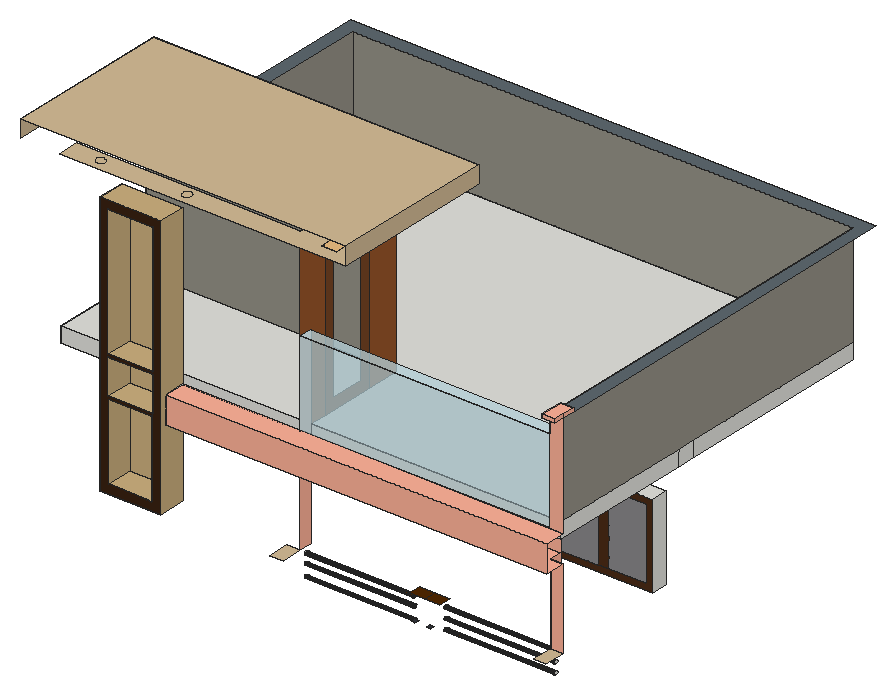
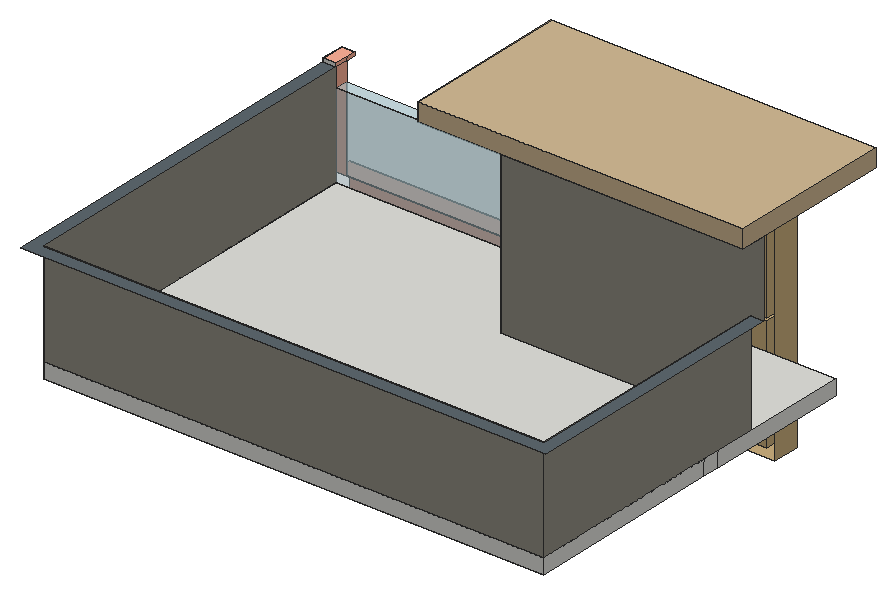
# SketchUp Ruby script. Lengths in inches.
U = 1.inch
M = Sketchup.active_model
def pt(a) = Geom::Point3d.new(a.map { |v| v * U })
def face(e, loops, mat)
  f = e.add_face(loops[0].map { |a| pt(a) })
  loops[1..].each { |l| e.add_face(l.map { |a| pt(a) }).erase! }
  f.material = f.back_material = mat if mat
  f
end
# faces: each face lists its corners as indices into pts; further lists are holes
def faces(e, pts, list, mat = nil) = list.each { |f| face(e, (f[0].is_a?(Array) ? f : [f]).map { |l| l.map { |i| pts[i] } }, mat) }
# xy, xz, yz: faces in a plane at the given z, y or x. An outline is a flat list of corners, or four numbers for a rectangle; further outlines are holes
def ring(l) = l.size == 4 ? [[l[0], l[1]], [l[2], l[1]], [l[2], l[3]], [l[0], l[3]]] : l.each_slice(2).to_a
def flat(e, list, mat, &to3) = list.each { |f| face(e, (f[0].is_a?(Array) ? f : [f]).map { |l| ring(l).map { |u, v| to3.(u, v) } }, mat) }
def xy(e, z, list, mat = nil) = flat(e, list, mat) { |x, y| [x, y, z] }
def xz(e, y, list, mat = nil) = flat(e, list, mat) { |x, z| [x, y, z] }
def yz(e, x, list, mat = nil) = flat(e, list, mat) { |y, z| [x, y, z] }
def lines(e, pts, list) = list.each { |a, b| e.add_line(pt(pts[a]), pt(pts[b])) }
# prism: a flat outline (further loops are holes) pulled along v
def prism(e, loops, v, mat = nil)
  f = face(e, loops, mat); d = Geom::Vector3d.new(v.map { |x| x * U })
  f.pushpull(f.normal.samedirection?(d) ? d.length : -d.length)
end
def box(e, o, s, mat = nil) = prism(e, [[o, [o[0] + s[0], o[1], o[2]], [o[0] + s[0], o[1] + s[1], o[2]], [o[0], o[1] + s[1], o[2]]]], [0, 0, s[2]], mat)
def at(x, y, z, deg = 0) = Geom::Transformation.translation(pt([x, y, z])) * Geom::Transformation.rotation(ORIGIN, Z_AXIS, deg.degrees)
def axes(o, x, y, z) = Geom::Transformation.new([*x, 0, *y, 0, *z, 0, *pt(o).to_a, 1])
def part(name) = M.definitions.add(name)
# library, detail: a bought-in or finely detailed component or shape, given as its bounding box
def library(name, o, s) = part(name).tap { |d| box(d.entities, o, s) }
def detail(e, o, s) = box(e.add_group.entities, o, s)
def put(e, d, t, mat = nil) = e.add_instance(d, t).tap { |i| i.material = mat if mat }
def group(e, t, mat = nil) = e.add_group.tap { |g| g.transformation = t; g.material = mat if mat }.entities
root = M.entities
M.materials.add("[Blinds Wood White]").color = [138, 137, 139]
M.materials.add("[Color B02]").color = [255, 178, 153]
M.materials.add("[Color C07]").color = [81, 40, 0]
M.materials.add("[Formica Beige]").color = [211, 187, 149]
M.materials.add("[Formica Graystone]").color = [149, 146, 135]
M.materials.add("[Formica Laminate Dark]").color = [50, 53, 60]
M.materials.add("[Formica Speckled Grey]").color = [94, 105, 111]
M.materials.add("[Translucent Glass Safety]").color = [204, 235, 244]
M.materials["[Translucent Glass Safety]"].alpha = 0.5
M.materials.add("[Wood Cherry Original]").color = [152, 86, 42]
M.materials.add("[Wood Floor Light]").color = [204, 176, 127]
M.materials.add("[Wood Veneer 01]").color = [76, 44, 23]
M.materials.add("[Wood Veneer 01]1").color = [58, 34, 18]
M.materials.add("[Wood Veneer 01]2").color = [120, 70, 37]
c1 = library("Group\#6",[-0.5,-0.5,-0.1],[13.21,13.21,0.2])
c2 = library("Group\#7",[-0.5,-0.5,-0.1],[13.21,13.21,0.2])
c3 = library("Group\#8",[-0.5,-0.5,-0.1],[13.21,13.21,0.2])
c4 = library("Group\#9",[-0.5,-0.5,-0.1],[13.21,13.21,0.2])
c5 = library("Group\#10",[-0.5,-0.5,-0.1],[13.21,13.21,0.2])
c6 = library("Group\#11",[-0.5,-0.5,-0.1],[13.21,13.21,0.2])
c7 = library("Group\#1",[-0.5,-0.5,-0.1],[10.625,10.625,0.2])
c8 = library("Group\#2",[-0.5,-0.5,-0.1],[10.625,10.625,0.2])
c9 = library("Group\#3",[-0.5,-0.5,-0.1],[10.625,10.625,0.2])
c10 = library("Group\#4",[-0.5,-0.5,-0.1],[10.625,10.625,0.2])
c11 = library("Group\#5",[-0.5,-0.5,-0.1],[10.625,10.625,0.2])
xy(root,43.38,[[349.875,213.0625,418,224.66]])
xy(root,49.9,[[342.13,97.98,344.57,100.8],[352.82,97.98,355.26,100.8]],"[Formica Laminate Dark]")
xy(root,64.77,[[338.39,100.8,348.76,109.8],[348.76,100.8,359.13,109.8]],"[Color C07]")
xy(root,64.77,[[252.91,86.05,262.24,100.8],[436.45,86.05,445.45,100.8]],"[Formica Beige]")
xy(root,66.71,[[137.86,81.92,180.23,100.8]],"[Wood Floor Light]")
xy(root,72.68,[[143.82,81.92,174.27,100.8]],"[Wood Floor Light]")
xy(root,101.95,[[349.875,213.0625,418,224.66]])
xy(root,113.3,[[266,213.0625,320.78,224.66]])
xy(root,120.54,[[180.23,86.42,180.23,100.8,262.24,100.8,262.24,109.8,436.45,109.8,436.45,100.8,445.45,100.8,445.45,86.42]],"[Color B02]")
xy(root,126.03,[[143.82,81.92,174.27,100.8]],"[Wood Floor Light]")
xy(root,127.75,[[143.49,81.92,174.6,100.8]],"[Wood Floor Light]")
xy(root,129,[[88.02,213.0625,436.45,224.66],[88.02,224.66,436.45,364.42]])
xy(root,129,[[88.02,109.8,436.45,213.0625]],"[Color B02]")
xy(root,139.625,[[262.24,109.8,436.45,109.8,436.45,364.42,88.02,364.42,88.02,184.36,262.24,184.36],[88.02,109.8,262.24,184.36]])
xy(root,139.625,[[180.23,86.42,445.45,100.8]],"[Color B02]")
xy(root,152.24,[[143.49,81.92,174.6,100.8]],"[Wood Floor Light]")
xy(root,153.94,[[143.49,81.92,174.6,100.8]],"[Wood Floor Light]")
xy(root,198.5625,[[262.24,100.8,436.24,100.8,436.45,109.8,262.24,109.8]],"[Translucent Glass Safety]")
xy(root,211.625,[[436.24,93.61,445.45,100.8],[436.24,100.8,436.45,109.8,445.45,109.8,445.45,100.8]])
xy(root,211.625,[[436.45,109.8,445.45,109.8,445.45,373.42,79.02,373.42,79.02,184.36,88.02,184.36,88.02,364.42,436.45,364.42]],"[Formica Speckled Grey]")
xy(root,214.0625,[[436.24,93.61,445.45,93.61,445.45,109.8,436.45,109.8,436.24,100.8]],"[Color B02]")
xy(root,244.36,[[143.49,81.92,174.6,100.8]],"[Wood Floor Light]")
xy(root,250,[[137.86,81.92,180.23,100.8]],"[Wood Floor Light]")
xy(root,264.08,[[[106.35,86.05,106.35,100.8,262.24,100.8,262.24,184.36,79.02,184.36,79.02,201.92,305.61,201.92,305.61,86.05],[128.96,90.32,129.87,90.43,130.71,90.78,131.43,91.34,131.99,92.07,132.34,92.91,132.46,93.82,132.34,94.72,131.99,95.57,131.43,96.29,130.71,96.85,129.87,97.2,128.96,97.32,128.05,97.2,127.21,96.85,126.49,96.29,125.93,95.57,125.58,94.72,125.46,93.82,125.58,92.91,125.93,92.07,126.49,91.34,127.21,90.78,128.05,90.43],[189.02,90.32,189.93,90.43,190.77,90.78,191.5,91.34,192.05,92.07,192.4,92.91,192.52,93.82,192.4,94.72,192.05,95.57,191.5,96.29,190.77,96.85,189.93,97.2,189.02,97.32,188.12,97.2,187.27,96.85,186.55,96.29,185.99,95.57,185.64,94.72,185.52,93.82,185.64,92.91,185.99,92.07,186.55,91.34,187.27,90.78,188.12,90.43]],[128.96,90.32,128.05,90.43,127.21,90.78,126.49,91.34,125.93,92.07,125.58,92.91,125.46,93.82,125.58,94.72,125.93,95.57,126.49,96.29,127.21,96.85,128.05,97.2,128.96,97.32,129.87,97.2,130.71,96.85,131.43,96.29,131.99,95.57,132.34,94.72,132.46,93.82,132.34,92.91,131.99,92.07,131.43,91.34,130.71,90.78,129.87,90.43],[189.02,90.32,188.12,90.43,187.27,90.78,186.55,91.34,185.99,92.07,185.64,92.91,185.52,93.82,185.64,94.72,185.99,95.57,186.55,96.29,187.27,96.85,188.12,97.2,189.02,97.32,189.93,97.2,190.77,96.85,191.5,96.29,192.05,95.57,192.4,94.72,192.52,93.82,192.4,92.91,192.05,92.07,191.5,91.34,190.77,90.78,189.93,90.43]],"[Formica Beige]")
xy(root,276.4375,[[79.02,86.05,305.61,201.92]],"[Formica Beige]")
xz(root,81.92,[[[137.86,66.71,180.23,250],[143.82,72.68,143.82,116.16,143.49,127.75,143.49,244.36,174.6,244.36,174.6,153.94,143.49,153.94,143.49,152.24,174.6,152.24,174.6,127.75,143.49,127.75,143.82,116.16,143.82,126.03,174.27,126.03,174.27,72.68]]],"[Wood Veneer 01]1")
xz(root,86.42,[[180.23,120.54,445.45,139.625]],"[Color B02]")
xz(root,93.61,[[436.24,211.625,445.45,214.0625]],"[Color B02]")
xz(root,100.8,[[180.23,120.54,262.24,139.625]])
xz(root,100.8,[[436.45,64.77,445.45,120.54],[436.24,139.625,445.45,211.625]],"[Color B02]")
xz(root,100.8,[[262.24,139.625,436.24,198.5625]],"[Translucent Glass Safety]")
xz(root,100.8,[[143.82,72.68,174.27,126.03],[143.49,127.75,174.6,152.24],[143.49,153.94,174.6,244.36]],"[Wood Floor Light]")
xz(root,109.8,[[88.02,129,262.24,139.625],[262.24,129,436.45,139.625],[436.45,211.625,445.45,214.0625]])
xz(root,109.8,[[262.24,120.54,436.45,129]],"[Color B02]")
xz(root,109.8,[[262.24,139.625,436.45,198.5625]],"[Translucent Glass Safety]")
xz(root,184.36,[[88.02,139.625,88.02,211.625,79.02,211.625,79.02,264.08,262.24,264.08,262.24,139.625]],"[Formica Graystone]")
xz(root,201.92,[[79.02,264.08,305.61,276.4375]],"[Formica Beige]")
xz(root,213.0625,[[354.23,47.73,379.68,97.59],[387.32,47.73,413.65,97.59]],"[Blinds Wood White]")
xz(root,213.0625,[[275.21,50.38,279.02,74.76]],"[Wood Floor Light]")
xz(root,213.0625,[[[349.875,43.38,418,101.95],[354.23,47.73,413.65,97.59]],[379.68,47.73,387.32,97.59]],"[Wood Veneer 01]")
xz(root,364.42,[[88.02,129,436.45,139.625]])
xz(root,364.42,[[88.02,139.625,436.45,211.625]],"[Formica Graystone]")
yz(root,79.02,[[86.05,264.08,201.92,276.4375]],"[Formica Beige]")
yz(root,88.02,[[109.8,129,213.0625,139.625],[213.0625,129,224.66,139.625],[224.66,129,364.42,139.625]])
yz(root,88.02,[[184.36,139.625,364.42,211.625]],"[Formica Graystone]")
yz(root,137.86,[[81.92,66.71,100.8,250]],"[Wood Floor Light]")
yz(root,143.49,[[81.92,127.75,100.8,152.24],[81.92,153.94,100.8,244.36]],"[Wood Floor Light]")
yz(root,143.82,[[81.92,72.68,100.8,126.03]],"[Wood Floor Light]")
yz(root,174.27,[[81.92,72.68,100.8,126.03]],"[Wood Floor Light]")
yz(root,174.6,[[81.92,127.75,100.8,152.24],[81.92,153.94,100.8,244.36]],"[Wood Floor Light]")
yz(root,180.23,[[86.42,120.54,100.8,122.12],[86.42,122.12,100.8,139.625]])
yz(root,180.23,[[81.92,66.71,100.8,66.71,100.8,120.54,86.42,120.54,86.42,139.625,100.8,139.625,100.8,250,81.92,250]],"[Wood Floor Light]")
yz(root,262.24,[[105.68,45.42,105.43,45.46,105.18,45.56,104.98,45.72,104.82,45.92,104.72,46.17,104.68,46.42,104.72,46.68,104.82,46.92,104.98,47.13,105.18,47.29,105.43,47.39,105.68,47.42,105.94,47.39,106.18,47.29,106.39,47.13,106.55,46.92,106.65,46.68,106.68,46.42,106.65,46.17,106.55,45.92,106.39,45.72,106.18,45.56,105.94,45.46],[105.68,53.61,105.43,53.65,105.18,53.75,104.98,53.9,104.82,54.11,104.72,54.35,104.68,54.61,104.72,54.87,104.82,55.11,104.98,55.32,105.18,55.48,105.43,55.58,105.68,55.61,105.94,55.58,106.18,55.48,106.39,55.32,106.55,55.11,106.65,54.87,106.68,54.61,106.65,54.35,106.55,54.11,106.39,53.9,106.18,53.75,105.94,53.65],[105.68,60.05,105.43,60.08,105.18,60.18,104.98,60.34,104.82,60.55,104.72,60.79,104.68,61.05,104.72,61.31,104.82,61.55,104.98,61.76,105.18,61.92,105.43,62.02,105.68,62.05,105.94,62.02,106.18,61.92,106.39,61.76,106.55,61.55,106.65,61.31,106.68,61.05,106.65,60.79,106.55,60.55,106.39,60.34,106.18,60.18,105.94,60.08],[100.8,120.54,109.8,198.5625]])
yz(root,262.24,[[100.8,64.77,109.8,120.54]],"[Color B02]")
yz(root,262.24,[[109.8,139.625,121.85,139.625,121.85,239.5625,161.15,239.5625,161.15,139.625,184.36,139.625,184.36,264.08,100.8,264.08,100.8,198.5625,109.8,198.5625]],"[Wood Cherry Original]")
yz(root,262.24,[[[121.85,139.625,161.15,239.5625],[129.39,147.17,153.61,232.02]]],"[Wood Veneer 01]2")
yz(root,305.61,[[86.05,264.08,201.92,276.4375]],"[Formica Beige]")
yz(root,349.875,[[213.0625,43.38,224.66,101.95]])
yz(root,418,[[213.0625,43.38,224.66,101.95]])
yz(root,436.24,[[93.61,211.625,100.8,214.0625]],"[Color B02]")
yz(root,436.45,[[106.01,46.23,106.27,46.26,106.51,46.36,106.72,46.52,106.875,46.73,106.98,46.97,107.01,47.23,106.98,47.49,106.875,47.73,106.72,47.9375,106.51,48.1,106.27,48.2,106.01,48.23,105.75,48.2,105.51,48.1,105.3,47.9375,105.14,47.73,105.04,47.49,105.01,47.23,105.04,46.97,105.14,46.73,105.3,46.52,105.51,46.36,105.75,46.26],[106.01,53.17,106.27,53.2,106.51,53.3,106.72,53.46,106.875,53.67,106.98,53.91,107.01,54.17,106.98,54.43,106.875,54.67,106.72,54.875,106.51,55.03,106.27,55.13,106.01,55.17,105.75,55.13,105.51,55.03,105.3,54.875,105.14,54.67,105.04,54.43,105.01,54.17,105.04,53.91,105.14,53.67,105.3,53.46,105.51,53.3,105.75,53.2],[106.01,60.17,106.27,60.2,106.51,60.3,106.72,60.46,106.875,60.67,106.98,60.91,107.01,61.17,106.98,61.43,106.875,61.67,106.72,61.875,106.51,62.03,106.27,62.13,106.01,62.17,105.75,62.13,105.51,62.03,105.3,61.875,105.14,61.67,105.04,61.43,105.01,61.17,105.04,60.91,105.14,60.67,105.3,60.46,105.51,60.3,105.75,60.2],[109.8,129,213.0625,139.625],[213.0625,129,224.66,139.625],
  [224.66,129,364.42,139.625]])
yz(root,436.45,[[100.8,64.77,109.8,120.54]],"[Color B02]")
yz(root,436.45,[[109.8,139.625,364.42,211.625]],"[Formica Graystone]")
yz(root,445.45,[[93.61,211.625,100.8,214.0625],[100.8,211.625,109.8,214.0625]],"[Color B02]")
p = [[262.24,105.43,45.46],[262.24,105.68,45.42],[338.39,105.68,45.42],[338.39,105.43,45.46],[262.24,105.94,45.46],[338.39,105.94,45.46],
  [262.24,105.18,45.56],[338.39,105.18,45.56],[262.24,106.18,45.56],[338.39,106.18,45.56],[262.24,104.98,45.72],[338.39,104.98,45.72],
  [262.24,106.39,45.72],[338.39,106.39,45.72],[262.24,104.82,45.92],[338.39,104.82,45.92],[262.24,106.55,45.92],[338.39,106.55,45.92],
  [262.24,104.72,46.17],[338.39,104.72,46.17],[262.24,106.65,46.17],[338.39,106.65,46.17],[262.24,104.68,46.42],[338.39,104.68,46.42],
  [436.45,106.01,46.23],[436.45,105.75,46.26],[359.13,105.75,46.26],[359.13,106.01,46.23],[436.45,106.27,46.26],[359.13,106.27,46.26],
  [262.24,106.68,46.42],[338.39,106.68,46.42],[436.45,105.51,46.36],[359.13,105.51,46.36],[436.45,106.51,46.36],[359.13,106.51,46.36],
  [262.24,104.72,46.68],[338.39,104.72,46.68],[436.45,105.3,46.52],[359.13,105.3,46.52],[436.45,106.72,46.52],[359.13,106.72,46.52],
  [262.24,106.65,46.68],[338.39,106.65,46.68],[436.45,105.14,46.73],[359.13,105.14,46.73],[436.45,106.875,46.73],[359.13,106.875,46.73],
  [262.24,104.82,46.92],[338.39,104.82,46.92],[436.45,105.04,46.97],[359.13,105.04,46.97],[262.24,106.55,46.92],[338.39,106.55,46.92],
  [436.45,106.98,46.97],[359.13,106.98,46.97],[262.24,104.98,47.13],[338.39,104.98,47.13],[262.24,106.39,47.13],[338.39,106.39,47.13],
  [436.45,105.01,47.23],[359.13,105.01,47.23],[436.45,107.01,47.23],[359.13,107.01,47.23],[262.24,105.18,47.29],[338.39,105.18,47.29],
  [262.24,106.18,47.29],[338.39,106.18,47.29],[436.45,105.04,47.49],[359.13,105.04,47.49],[436.45,106.98,47.49],[359.13,106.98,47.49],
  [262.24,105.43,47.39],[338.39,105.43,47.39],[262.24,105.94,47.39],[338.39,105.94,47.39],[262.24,105.68,47.42],[338.39,105.68,47.42],
  [436.45,105.14,47.73],[359.13,105.14,47.73],[436.45,106.875,47.73],[359.13,106.875,47.73],[436.45,105.3,47.9375],[359.13,105.3,47.9375],
  [436.45,106.72,47.9375],[359.13,106.72,47.9375],[436.45,105.51,48.1],[359.13,105.51,48.1],[436.45,106.51,48.1],[359.13,106.51,48.1],
  [436.45,105.75,48.2],[359.13,105.75,48.2],[436.45,106.27,48.2],[359.13,106.27,48.2],[436.45,106.01,48.23],[359.13,106.01,48.23],
  [436.45,105.75,53.2],[436.45,105.51,53.3],[359.13,105.51,53.3],[359.13,105.75,53.2],[436.45,106.01,53.17],[359.13,106.01,53.17],
  [436.45,106.27,53.2],[359.13,106.27,53.2],[436.45,106.51,53.3],[359.13,106.51,53.3],[436.45,105.3,53.46],[359.13,105.3,53.46],
  [436.45,106.72,53.46],[359.13,106.72,53.46],[436.45,105.14,53.67],[359.13,105.14,53.67],[436.45,106.875,53.67],[359.13,106.875,53.67],
  [262.24,105.18,53.75],[262.24,105.43,53.65],[338.39,105.43,53.65],[338.39,105.18,53.75],[262.24,105.68,53.61],[338.39,105.68,53.61],
  [262.24,105.94,53.65],[338.39,105.94,53.65],[262.24,106.18,53.75],[338.39,106.18,53.75],[262.24,104.98,53.9],[338.39,104.98,53.9],
  [436.45,105.04,53.91],[359.13,105.04,53.91],[262.24,106.39,53.9],[338.39,106.39,53.9],[436.45,106.98,53.91],[359.13,106.98,53.91],
  [262.24,104.82,54.11],[338.39,104.82,54.11],[436.45,105.01,54.17],[359.13,105.01,54.17],[262.24,106.55,54.11],[338.39,106.55,54.11],
  [436.45,107.01,54.17],[359.13,107.01,54.17],[262.24,104.72,54.35],[338.39,104.72,54.35],[262.24,106.65,54.35],[338.39,106.65,54.35],
  [436.45,105.04,54.43],[359.13,105.04,54.43],[436.45,106.98,54.43],[359.13,106.98,54.43],[262.24,104.68,54.61],[338.39,104.68,54.61],
  [436.45,105.14,54.67],[359.13,105.14,54.67],[262.24,106.68,54.61],[338.39,106.68,54.61],[436.45,106.875,54.67],[359.13,106.875,54.67],
  [262.24,104.72,54.87],[338.39,104.72,54.87],[262.24,106.65,54.87],[338.39,106.65,54.87],[436.45,105.3,54.875],[359.13,105.3,54.875],
  [436.45,106.72,54.875],[359.13,106.72,54.875],[262.24,104.82,55.11],[338.39,104.82,55.11],[436.45,105.51,55.03],[359.13,105.51,55.03],
  [436.45,106.51,55.03],[359.13,106.51,55.03],[262.24,106.55,55.11],[338.39,106.55,55.11],[436.45,105.75,55.13],[359.13,105.75,55.13],
  [436.45,106.27,55.13],[359.13,106.27,55.13],[262.24,104.98,55.32],[338.39,104.98,55.32],[436.45,106.01,55.17],[359.13,106.01,55.17],
  [262.24,106.39,55.32],[338.39,106.39,55.32],[262.24,105.18,55.48],[338.39,105.18,55.48],[262.24,106.18,55.48],[338.39,106.18,55.48],
  [262.24,105.43,55.58],[338.39,105.43,55.58],[262.24,105.94,55.58],[338.39,105.94,55.58],[262.24,105.68,55.61],[338.39,105.68,55.61],
  [262.24,105.43,60.08],[262.24,105.68,60.05],[338.39,105.68,60.05],[338.39,105.43,60.08],[262.24,105.94,60.08],[338.39,105.94,60.08],
  [262.24,105.18,60.18],[338.39,105.18,60.18],[262.24,106.18,60.18],[338.39,106.18,60.18],[262.24,104.98,60.34],[338.39,104.98,60.34],
  [436.45,105.75,60.2],[436.45,105.51,60.3],[359.13,105.51,60.3],[359.13,105.75,60.2],[436.45,106.01,60.17],[359.13,106.01,60.17],
  [436.45,106.27,60.2],[359.13,106.27,60.2],[262.24,106.39,60.34],[338.39,106.39,60.34],[436.45,106.51,60.3],[359.13,106.51,60.3],
  [262.24,104.82,60.55],[338.39,104.82,60.55],[436.45,105.3,60.46],[359.13,105.3,60.46],[262.24,106.55,60.55],[338.39,106.55,60.55],
  [436.45,106.72,60.46],[359.13,106.72,60.46],[262.24,104.72,60.79],[338.39,104.72,60.79],[436.45,105.14,60.67],[359.13,105.14,60.67],
  [262.24,106.65,60.79],[338.39,106.65,60.79],[436.45,106.875,60.67],[359.13,106.875,60.67],[436.45,105.04,60.91],[359.13,105.04,60.91],
  [436.45,106.98,60.91],[359.13,106.98,60.91],[262.24,104.68,61.05],[338.39,104.68,61.05],[262.24,106.68,61.05],[338.39,106.68,61.05],
  [436.45,105.01,61.17],[359.13,105.01,61.17],[436.45,107.01,61.17],[359.13,107.01,61.17],[262.24,104.72,61.31],[338.39,104.72,61.31],
  [262.24,106.65,61.31],[338.39,106.65,61.31],[436.45,105.04,61.43],[359.13,105.04,61.43],[436.45,106.98,61.43],[359.13,106.98,61.43],
  [262.24,104.82,61.55],[338.39,104.82,61.55],[262.24,106.55,61.55],[338.39,106.55,61.55],[436.45,105.14,61.67],[359.13,105.14,61.67],
  [436.45,106.875,61.67],[359.13,106.875,61.67],[262.24,104.98,61.76],[338.39,104.98,61.76],[262.24,106.39,61.76],[338.39,106.39,61.76],
  [436.45,105.3,61.875],[359.13,105.3,61.875],[436.45,106.72,61.875],[359.13,106.72,61.875],[262.24,105.18,61.92],[338.39,105.18,61.92],
  [262.24,106.18,61.92],[338.39,106.18,61.92],[262.24,105.43,62.02],[338.39,105.43,62.02],[436.45,105.51,62.03],[359.13,105.51,62.03],
  [262.24,105.94,62.02],[338.39,105.94,62.02],[436.45,106.51,62.03],[359.13,106.51,62.03],[262.24,105.68,62.05],[338.39,105.68,62.05],
  [436.45,105.75,62.13],[359.13,105.75,62.13],[436.45,106.27,62.13],[359.13,106.27,62.13],[436.45,106.01,62.17],[359.13,106.01,62.17],
  [436.45,109.8,211.625],[436.45,109.8,198.5625],[436.24,100.8,198.5625],[436.24,100.8,211.625],[436.24,100.8,214.0625],[436.45,109.8,214.0625]]
faces(root,p,[[0,1,2,3],[1,4,5,2],[6,0,3,7],[4,8,9,5],[10,6,7,11],[8,12,13,9],[14,10,11,15],[12,16,17,13],
  [18,14,15,19],[16,20,21,17],[22,18,19,23],[24,25,26,27],[28,24,27,29],[20,30,31,21],[25,32,33,26],[34,28,29,35],
  [36,22,23,37],[32,38,39,33],[40,34,35,41],[30,42,43,31],[38,44,45,39],[46,40,41,47],[48,36,37,49],[44,50,51,45],
  [42,52,53,43],[54,46,47,55],[56,48,49,57],[52,58,59,53],[50,60,61,51],[62,54,55,63],[64,56,57,65],[58,66,67,59],
  [60,68,69,61],[70,62,63,71],[72,64,65,73],[66,74,75,67],[76,72,73,77],[74,76,77,75],[68,78,79,69],[80,70,71,81],
  [78,82,83,79],[84,80,81,85],[82,86,87,83],[88,84,85,89],[86,90,91,87],[92,88,89,93],[90,94,95,91],[94,92,93,95],
  [96,97,98,99],[100,96,99,101],[102,100,101,103],[104,102,103,105],[97,106,107,98],[108,104,105,109],[106,110,111,107],[112,108,109,113],
  [114,115,116,117],[115,118,119,116],[118,120,121,119],[120,122,123,121],[124,114,117,125],[110,126,127,111],[122,128,129,123],[130,112,113,131],
  [132,124,125,133],[126,134,135,127],[128,136,137,129],[138,130,131,139],[140,132,133,141],[136,142,143,137],[134,144,145,135],[146,138,139,147],
  [148,140,141,149],[144,150,151,145],[142,152,153,143],[154,146,147,155],[156,148,149,157],[152,158,159,153],[150,160,161,151],[162,154,155,163],
  [164,156,157,165],[160,166,167,161],[168,162,163,169],[158,170,171,159],[166,172,173,167],[174,168,169,175],[176,164,165,177],[172,178,179,173],
  [178,174,175,179],[170,180,181,171],[182,176,177,183],[180,184,185,181],[186,182,183,187],[184,188,189,185],[190,186,187,191],[188,190,191,189],
  [192,193,194,195],[193,196,197,194],[198,192,195,199],[196,200,201,197],[202,198,199,203],[204,205,206,207],[208,204,207,209],[210,208,209,211],
  [200,212,213,201],[214,210,211,215],[216,202,203,217],[205,218,219,206],[212,220,221,213],[222,214,215,223],[224,216,217,225],[218,226,227,219],
  [220,228,229,221],[230,222,223,231],[226,232,233,227],[234,230,231,235],[236,224,225,237],[228,238,239,229],[232,240,241,233],[242,234,235,243],
  [244,236,237,245],[238,246,247,239],[240,248,249,241],[250,242,243,251],[252,244,245,253],[246,254,255,247],[248,256,257,249],[258,250,251,259],
  [260,252,253,261],[254,262,263,255],[256,264,265,257],[266,258,259,267],[268,260,261,269],[262,270,271,263],[272,268,269,273],[264,274,275,265],
  [270,276,277,271],[278,266,267,279],[280,272,273,281],[274,282,283,275],[276,280,281,277],[284,278,279,285],[282,286,287,283],[286,284,285,287]],"[Color C07]")
faces(root,p,[[288,289,290,291],[288,291,292,293]],"[Color B02]")
put(root,c1,axes([293.01,132.9,129],[-1,0,0],[0,1,0],[0,0,-1]))
put(root,c2,axes([283.52,180.97,129],[-1,0,0],[0,1,0],[0,0,-1]))
put(root,c3,axes([354.26,132.9,129],[-1,0,0],[0,1,0],[0,0,-1]))
put(root,c4,axes([354.26,178.21,129],[-1,0,0],[0,1,0],[0,0,-1]))
put(root,c5,axes([415.95,132.9,129],[-1,0,0],[0,1,0],[0,0,-1]))
put(root,c6,axes([423.2,178.21,129],[-1,0,0],[0,1,0],[0,0,-1]))
put(root,c7,axes([291.52,95.74,264.08],[-1,0,0],[0,1,0],[0,0,-1]))
put(root,c8,axes([291.52,115.93,264.08],[-1,0,0],[0,1,0],[0,0,-1]))
put(root,c9,axes([291.52,135.24,264.08],[-1,0,0],[0,1,0],[0,0,-1]))
put(root,c10,axes([291.52,158.18,264.08],[-1,0,0],[0,1,0],[0,0,-1]))
put(root,c11,axes([291.52,182.05,264.08],[-1,0,0],[0,1,0],[0,0,-1]))
